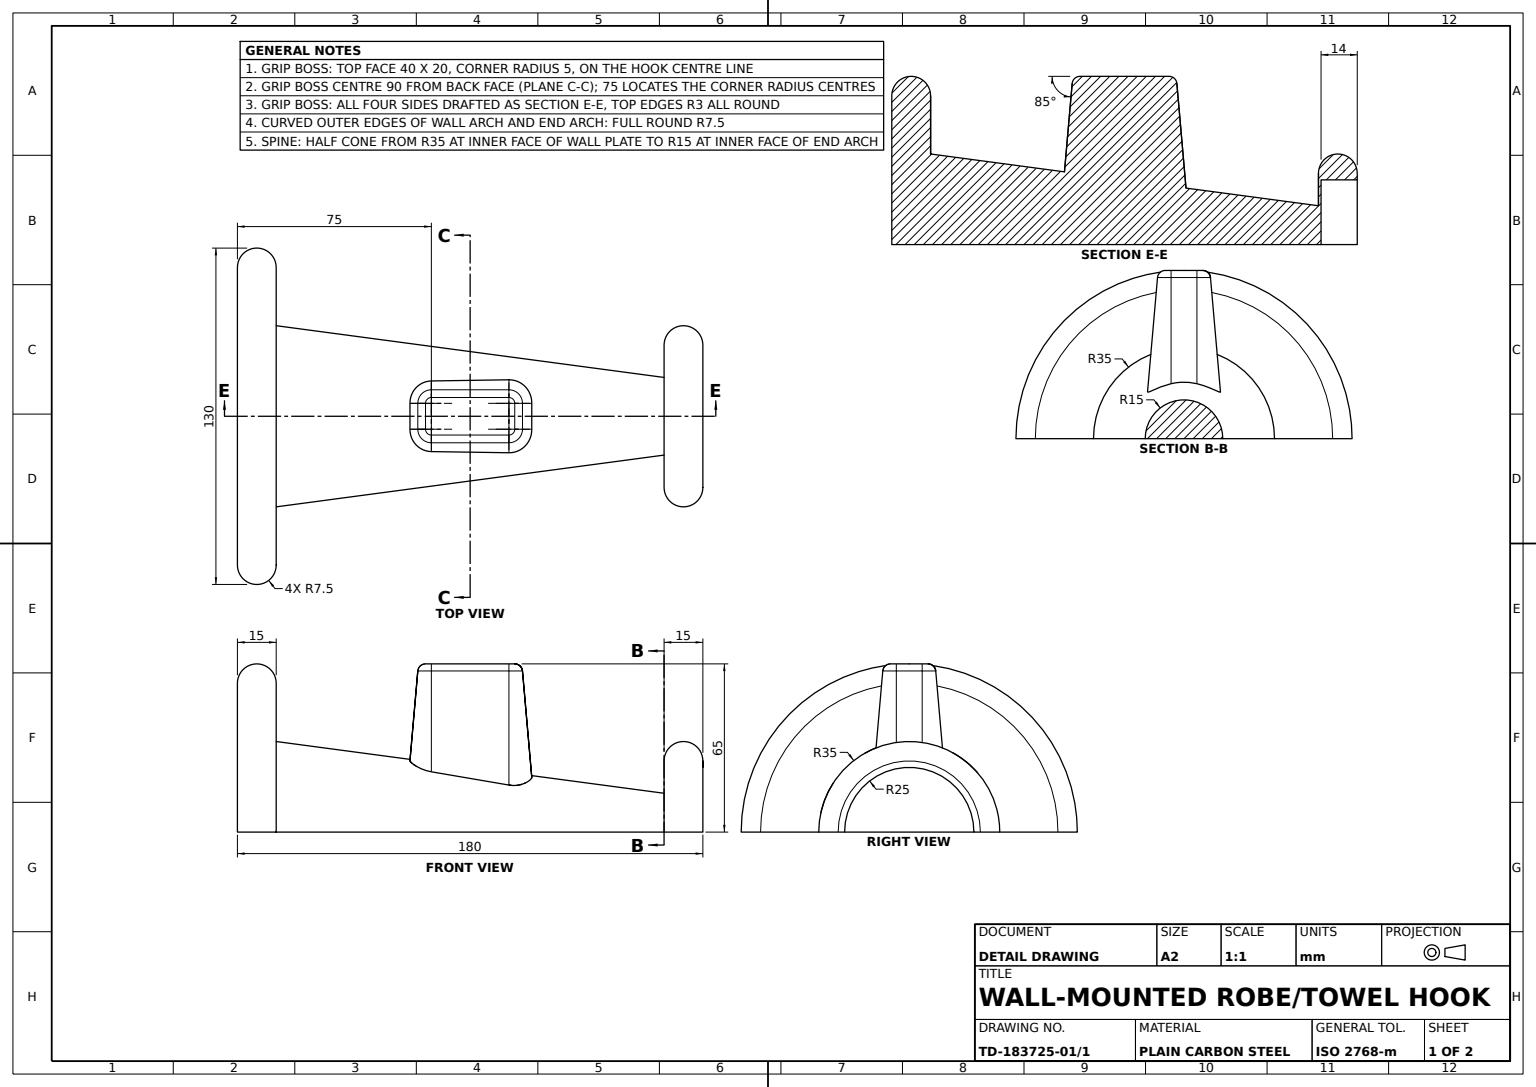
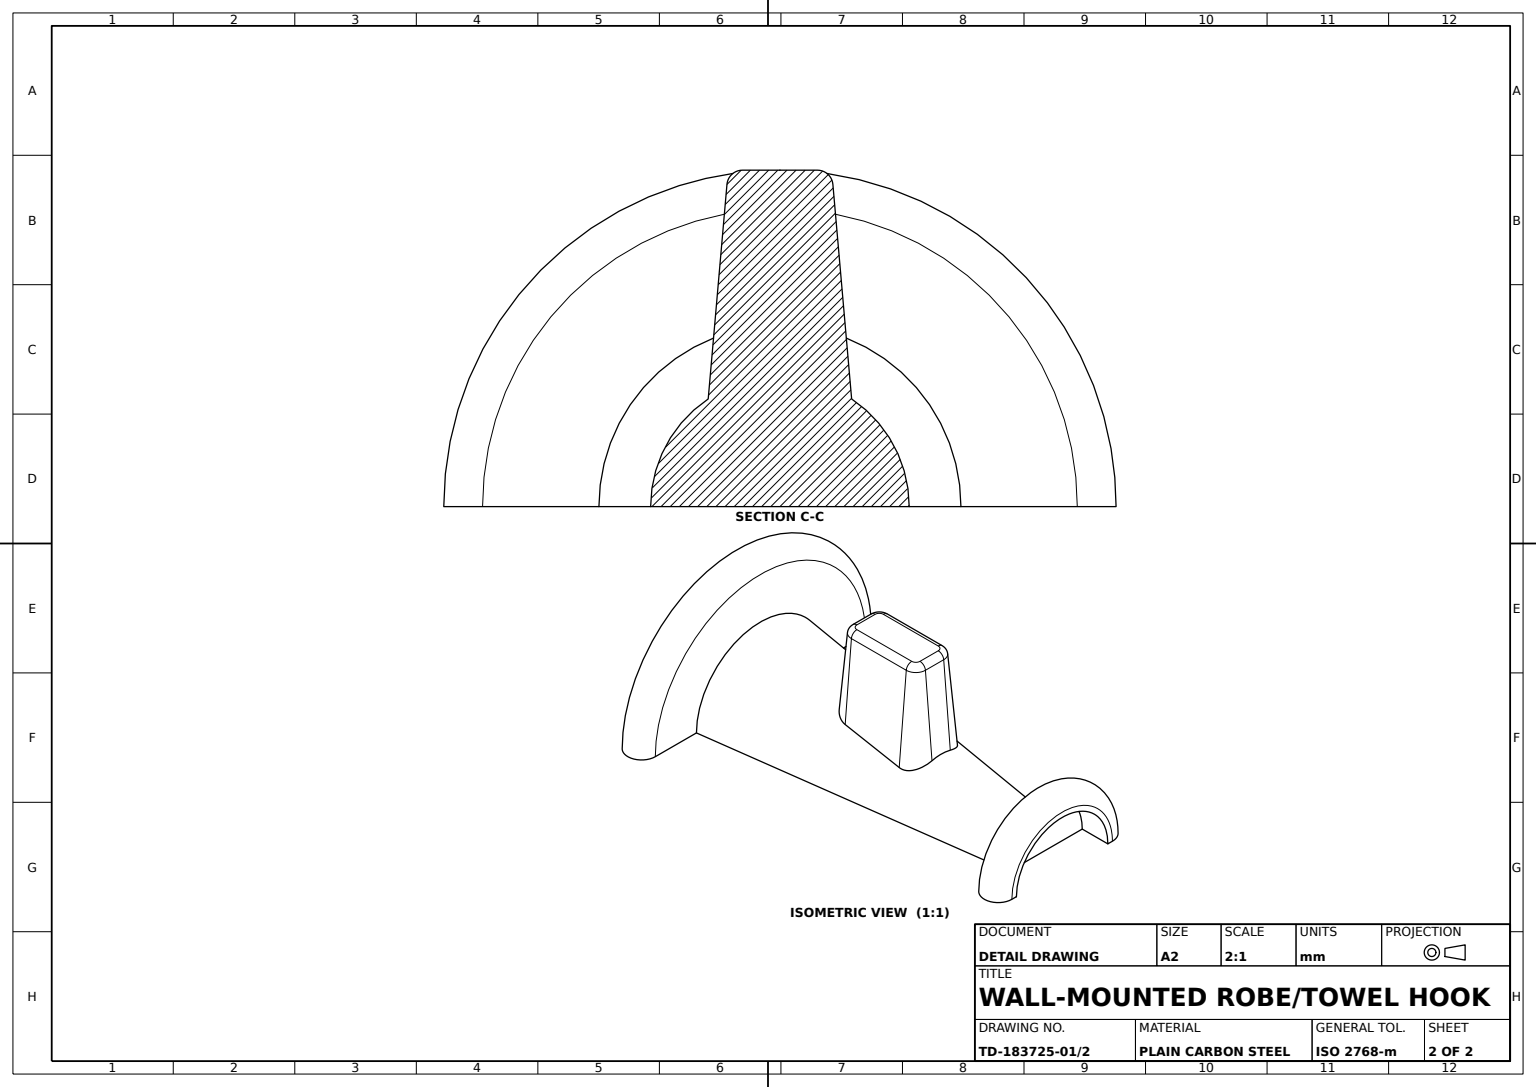
ISO-10303-21;
HEADER;
FILE_DESCRIPTION((''),'2;1');
FILE_NAME('','',(''),(''),'','','');
FILE_SCHEMA(('AUTOMOTIVE_DESIGN'));
ENDSEC;
DATA;
#1=APPLICATION_CONTEXT('');
#2=PRODUCT_CONTEXT('',#1,'mechanical');
#3=PRODUCT('','','',(#2));
#4=PRODUCT_DEFINITION_FORMATION('','',#3);
#5=PRODUCT_DEFINITION_CONTEXT('',#1,'design');
#6=PRODUCT_DEFINITION('','',#4,#5);
#7=PRODUCT_DEFINITION_SHAPE('','',#6);
#8=(LENGTH_UNIT()NAMED_UNIT(*)SI_UNIT(.MILLI.,.METRE.));
#9=(NAMED_UNIT(*)PLANE_ANGLE_UNIT()SI_UNIT($,.RADIAN.));
#10=(NAMED_UNIT(*)SI_UNIT($,.STERADIAN.)SOLID_ANGLE_UNIT());
#11=UNCERTAINTY_MEASURE_WITH_UNIT(LENGTH_MEASURE(1.E-05),#8,'distance_accuracy_value','');
#12=(GEOMETRIC_REPRESENTATION_CONTEXT(3)GLOBAL_UNCERTAINTY_ASSIGNED_CONTEXT((#11))GLOBAL_UNIT_ASSIGNED_CONTEXT((#8,#9,#10))REPRESENTATION_CONTEXT('',''));
#13=CARTESIAN_POINT('',(-90.,0.,-57.5));
#14=VERTEX_POINT('',#13);
#15=CARTESIAN_POINT('',(-90.,0.,57.5));
#16=VERTEX_POINT('',#15);
#17=CARTESIAN_POINT('',(-90.,0.,0.));
#18=DIRECTION('',(0.,0.,1.));
#19=VECTOR('',#18,1000.);
#20=LINE('',#17,#19);
#21=EDGE_CURVE('',#14,#16,#20,.T.);
#22=ORIENTED_EDGE('',*,*,#21,.T.);
#23=DIRECTION('',(-1.,0.,0.));
#24=AXIS2_PLACEMENT_3D('',#17,#23,#18);
#25=CIRCLE('',#24,57.5);
#26=EDGE_CURVE('',#16,#14,#25,.T.);
#27=ORIENTED_EDGE('',*,*,#26,.T.);
#28=EDGE_LOOP('',(#22,#27));
#29=FACE_OUTER_BOUND('',#28,.T.);
#30=PLANE('',#24);
#31=ADVANCED_FACE('',(#29),#30,.T.);
#32=CARTESIAN_POINT('',(15.,62.261467,-10.239591));
#33=VERTEX_POINT('',#32);
#34=CARTESIAN_POINT('',(20.239591,62.261467,-5.));
#35=VERTEX_POINT('',#34);
#36=CARTESIAN_POINT('',(15.,62.261467,-5.));
#37=DIRECTION('',(0.,-1.,0.));
#38=DIRECTION('',(0.,0.,-1.));
#39=AXIS2_PLACEMENT_3D('',#36,#37,#38);
#40=CIRCLE('',#39,5.239591);
#41=EDGE_CURVE('',#33,#35,#40,.T.);
#42=ORIENTED_EDGE('',*,*,#41,.F.);
#43=CARTESIAN_POINT('',(15.,65.,-7.251006));
#44=VERTEX_POINT('',#43);
#45=CARTESIAN_POINT('',(15.,62.,-7.251006));
#46=DIRECTION('',(1.,0.,0.));
#47=AXIS2_PLACEMENT_3D('',#45,#46,#38);
#48=CIRCLE('',#47,3.);
#49=EDGE_CURVE('',#33,#44,#48,.T.);
#50=ORIENTED_EDGE('',*,*,#49,.T.);
#51=CARTESIAN_POINT('',(17.251006,65.,-5.));
#52=VERTEX_POINT('',#51);
#53=CARTESIAN_POINT('',(15.,65.,-5.));
#54=DIRECTION('',(0.,1.,0.));
#55=AXIS2_PLACEMENT_3D('',#53,#54,#38);
#56=CIRCLE('',#55,2.251006);
#57=EDGE_CURVE('',#52,#44,#56,.T.);
#58=ORIENTED_EDGE('',*,*,#57,.F.);
#59=CARTESIAN_POINT('',(17.251006,62.,-5.));
#60=AXIS2_PLACEMENT_3D('',#59,#18,#46);
#61=CIRCLE('',#60,3.);
#62=EDGE_CURVE('',#35,#52,#61,.T.);
#63=ORIENTED_EDGE('',*,*,#62,.F.);
#64=EDGE_LOOP('',(#42,#50,#58,#63));
#65=FACE_OUTER_BOUND('',#64,.T.);
#66=CARTESIAN_POINT('',(15.,62.,-5.));
#67=AXIS2_PLACEMENT_3D('',#66,#37,#38);
#68=TOROIDAL_SURFACE('',#67,2.251006,3.);
#69=ADVANCED_FACE('',(#65),#68,.T.);
#70=CARTESIAN_POINT('',(-17.251006,65.,5.));
#71=VERTEX_POINT('',#70);
#72=CARTESIAN_POINT('',(-20.239591,62.261467,5.));
#73=VERTEX_POINT('',#72);
#74=CARTESIAN_POINT('',(-17.251006,62.,5.));
#75=AXIS2_PLACEMENT_3D('',#74,#18,#46);
#76=CIRCLE('',#75,3.);
#77=EDGE_CURVE('',#71,#73,#76,.T.);
#78=ORIENTED_EDGE('',*,*,#77,.F.);
#79=CARTESIAN_POINT('',(-17.251006,65.,-5.));
#80=VERTEX_POINT('',#79);
#81=LINE('',#70,#19);
#82=EDGE_CURVE('',#80,#71,#81,.T.);
#83=ORIENTED_EDGE('',*,*,#82,.F.);
#84=CARTESIAN_POINT('',(-20.239591,62.261467,-5.));
#85=VERTEX_POINT('',#84);
#86=CARTESIAN_POINT('',(-17.251006,62.,-5.));
#87=AXIS2_PLACEMENT_3D('',#86,#18,#46);
#88=CIRCLE('',#87,3.);
#89=EDGE_CURVE('',#80,#85,#88,.T.);
#90=ORIENTED_EDGE('',*,*,#89,.T.);
#91=VECTOR('',#38,1000.);
#92=LINE('',#84,#91);
#93=EDGE_CURVE('',#73,#85,#92,.T.);
#94=ORIENTED_EDGE('',*,*,#93,.F.);
#95=EDGE_LOOP('',(#78,#83,#90,#94));
#96=FACE_OUTER_BOUND('',#95,.T.);
#97=AXIS2_PLACEMENT_3D('',#86,#38,#23);
#98=CYLINDRICAL_SURFACE('',#97,3.);
#99=ADVANCED_FACE('',(#96),#98,.T.);
#100=CARTESIAN_POINT('',(76.,0.,-25.));
#101=VERTEX_POINT('',#100);
#102=CARTESIAN_POINT('',(76.,0.,25.));
#103=VERTEX_POINT('',#102);
#104=CARTESIAN_POINT('',(76.,0.,94.));
#105=LINE('',#104,#19);
#106=EDGE_CURVE('',#101,#103,#105,.T.);
#107=ORIENTED_EDGE('',*,*,#106,.F.);
#108=CARTESIAN_POINT('',(76.,0.,0.));
#109=AXIS2_PLACEMENT_3D('',#108,#46,#38);
#110=CIRCLE('',#109,25.);
#111=EDGE_CURVE('',#101,#103,#110,.T.);
#112=ORIENTED_EDGE('',*,*,#111,.T.);
#113=EDGE_LOOP('',(#107,#112));
#114=FACE_OUTER_BOUND('',#113,.T.);
#115=PLANE('',#109);
#116=ADVANCED_FACE('',(#114),#115,.T.);
#117=CARTESIAN_POINT('',(23.828296,21.24238,5.));
#118=VERTEX_POINT('',#117);
#119=CARTESIAN_POINT('',(20.239591,62.261467,5.));
#120=VERTEX_POINT('',#119);
#121=CARTESIAN_POINT('',(20.,65.,5.));
#122=DIRECTION('',(-0.087155743,0.996194698,0.));
#123=VECTOR('',#122,1000.);
#124=LINE('',#121,#123);
#125=EDGE_CURVE('',#118,#120,#124,.T.);
#126=ORIENTED_EDGE('',*,*,#125,.T.);
#127=CARTESIAN_POINT('',(15.,62.261467,10.239591));
#128=VERTEX_POINT('',#127);
#129=CARTESIAN_POINT('',(15.,62.261467,5.));
#130=AXIS2_PLACEMENT_3D('',#129,#37,#38);
#131=CIRCLE('',#130,5.239591);
#132=EDGE_CURVE('',#120,#128,#131,.T.);
#133=ORIENTED_EDGE('',*,*,#132,.T.);
#134=CARTESIAN_POINT('',(15.,18.173632,14.096776));
#135=VERTEX_POINT('',#134);
#136=CARTESIAN_POINT('',(15.,65.,10.));
#137=DIRECTION('',(0.,0.996194698,-0.087155743));
#138=VECTOR('',#137,1000.);
#139=LINE('',#136,#138);
#140=EDGE_CURVE('',#135,#128,#139,.T.);
#141=ORIENTED_EDGE('',*,*,#140,.F.);
#142=CARTESIAN_POINT('',(23.840601,21.101725,5.590409));
#143=CARTESIAN_POINT('',(23.795702,20.944319,6.174844));
#144=CARTESIAN_POINT('',(23.643977,20.683423,7.042667));
#145=CARTESIAN_POINT('',(23.579195,20.592513,7.329711));
#146=CARTESIAN_POINT('',(23.424423,20.406792,7.889331));
#147=CARTESIAN_POINT('',(23.334202,20.311543,8.163393));
#148=CARTESIAN_POINT('',(23.128661,20.117169,8.700562));
#149=CARTESIAN_POINT('',(23.013343,20.018041,8.963668));
#150=CARTESIAN_POINT('',(22.757306,19.816981,9.479197));
#151=CARTESIAN_POINT('',(22.615811,19.714543,9.73281));
#152=CARTESIAN_POINT('',(22.157707,19.409162,10.467784));
#153=CARTESIAN_POINT('',(21.809445,19.208631,10.922403));
#154=CARTESIAN_POINT('',(21.220199,18.923437,11.553938));
#155=CARTESIAN_POINT('',(21.01254,18.831012,11.755982));
#156=CARTESIAN_POINT('',(20.572849,18.654017,12.142651));
#157=CARTESIAN_POINT('',(20.340224,18.569371,12.327468));
#158=CARTESIAN_POINT('',(19.619318,18.337421,12.842278));
#159=CARTESIAN_POINT('',(19.103668,18.20966,13.137737));
#160=CARTESIAN_POINT('',(18.269214,18.077938,13.503422));
#161=CARTESIAN_POINT('',(17.98184,18.04451,13.611482));
#162=CARTESIAN_POINT('',(17.403424,18.002399,13.794297));
#163=CARTESIAN_POINT('',(17.110364,17.993364,13.869986));
#164=CARTESIAN_POINT('',(16.516526,18.000652,13.989928));
#165=CARTESIAN_POINT('',(16.215749,18.016974,14.034185));
#166=CARTESIAN_POINT('',(15.606218,18.076326,14.09024));
#167=CARTESIAN_POINT('',(15.300917,18.119158,14.101542));
#168=B_SPLINE_CURVE_WITH_KNOTS('',3,(#117,#142,#143,#144,#145,#146,#147,#148,#149,#150,#151,#152,#153,#154,#155,#156,#157,#158,#159,#160,#161,#162,#163,#164,#165,#166,#167,#134),.UNSPECIFIED.,.F.,.F.,(4,2,2,2,2,2,2,2,2,2,2,2,2,4),(0.001090919,0.002909668,0.003819042,0.004728417,0.005637791,0.006547165,0.008365914,0.009275289,0.010184663,0.012003412,0.012912786,0.013822161,0.014731535,0.01564091),.UNSPECIFIED.);
#169=EDGE_CURVE('',#118,#135,#168,.T.);
#170=ORIENTED_EDGE('',*,*,#169,.F.);
#171=EDGE_LOOP('',(#126,#133,#141,#170));
#172=FACE_OUTER_BOUND('',#171,.T.);
#173=CARTESIAN_POINT('',(15.,65.,5.));
#174=AXIS2_PLACEMENT_3D('',#173,#37,#18);
#175=CONICAL_SURFACE('',#174,5.,0.087266463);
#176=ADVANCED_FACE('',(#172),#175,.T.);
#177=CARTESIAN_POINT('',(90.,0.,-25.));
#178=VERTEX_POINT('',#177);
#179=CARTESIAN_POINT('',(90.,0.,25.));
#180=VERTEX_POINT('',#179);
#181=CARTESIAN_POINT('',(90.,0.,0.));
#182=AXIS2_PLACEMENT_3D('',#181,#46,#38);
#183=CIRCLE('',#182,25.);
#184=EDGE_CURVE('',#178,#180,#183,.T.);
#185=ORIENTED_EDGE('',*,*,#184,.T.);
#186=VECTOR('',#23,1000.);
#187=LINE('',#102,#186);
#188=EDGE_CURVE('',#180,#103,#187,.T.);
#189=ORIENTED_EDGE('',*,*,#188,.T.);
#190=ORIENTED_EDGE('',*,*,#111,.F.);
#191=VECTOR('',#46,1000.);
#192=LINE('',#100,#191);
#193=EDGE_CURVE('',#101,#178,#192,.T.);
#194=ORIENTED_EDGE('',*,*,#193,.T.);
#195=EDGE_LOOP('',(#185,#189,#190,#194));
#196=FACE_OUTER_BOUND('',#195,.T.);
#197=CYLINDRICAL_SURFACE('',#109,25.);
#198=ADVANCED_FACE('',(#196),#197,.F.);
#199=CARTESIAN_POINT('',(-75.,0.,57.5));
#200=VERTEX_POINT('',#199);
#201=CARTESIAN_POINT('',(-75.,0.,-57.5));
#202=VERTEX_POINT('',#201);
#203=CARTESIAN_POINT('',(-75.,0.,0.));
#204=AXIS2_PLACEMENT_3D('',#203,#23,#18);
#205=CIRCLE('',#204,57.5);
#206=EDGE_CURVE('',#200,#202,#205,.T.);
#207=ORIENTED_EDGE('',*,*,#206,.T.);
#208=CARTESIAN_POINT('',(-82.5,0.,-57.5));
#209=AXIS2_PLACEMENT_3D('',#208,#37,#38);
#210=CIRCLE('',#209,7.5);
#211=EDGE_CURVE('',#14,#202,#210,.T.);
#212=ORIENTED_EDGE('',*,*,#211,.F.);
#213=ORIENTED_EDGE('',*,*,#26,.F.);
#214=CARTESIAN_POINT('',(-82.5,0.,57.5));
#215=AXIS2_PLACEMENT_3D('',#214,#37,#38);
#216=CIRCLE('',#215,7.5);
#217=EDGE_CURVE('',#200,#16,#216,.T.);
#218=ORIENTED_EDGE('',*,*,#217,.F.);
#219=EDGE_LOOP('',(#207,#212,#213,#218));
#220=FACE_OUTER_BOUND('',#219,.T.);
#221=CARTESIAN_POINT('',(-82.5,0.,0.));
#222=AXIS2_PLACEMENT_3D('',#221,#23,#18);
#223=TOROIDAL_SURFACE('',#222,57.5,7.5);
#224=ADVANCED_FACE('',(#220),#223,.T.);
#225=CARTESIAN_POINT('',(-15.,23.296257,13.648605));
#226=VERTEX_POINT('',#225);
#227=CARTESIAN_POINT('',(-23.267357,27.653934,5.));
#228=VERTEX_POINT('',#227);
#229=CARTESIAN_POINT('',(-15.286863,23.342981,13.644517));
#230=CARTESIAN_POINT('',(-15.571632,23.39812,13.625462));
#231=CARTESIAN_POINT('',(-16.13718,23.524275,13.55813));
#232=CARTESIAN_POINT('',(-16.419535,23.595752,13.509462));
#233=CARTESIAN_POINT('',(-17.24849,23.829231,13.322204));
#234=CARTESIAN_POINT('',(-17.773834,24.008665,13.144495));
#235=CARTESIAN_POINT('',(-18.526695,24.303572,12.805119));
#236=CARTESIAN_POINT('',(-18.772818,24.406707,12.679069));
#237=CARTESIAN_POINT('',(-19.247498,24.617633,12.405792));
#238=CARTESIAN_POINT('',(-19.475861,24.725257,12.258861));
#239=CARTESIAN_POINT('',(-20.135824,25.052517,11.788166));
#240=CARTESIAN_POINT('',(-20.542582,25.276497,11.43483));
#241=CARTESIAN_POINT('',(-21.291765,25.726959,10.645748));
#242=CARTESIAN_POINT('',(-21.623823,25.947177,10.220874));
#243=CARTESIAN_POINT('',(-22.060957,26.264462,9.537608));
#244=CARTESIAN_POINT('',(-22.196427,26.36806,9.302129));
#245=CARTESIAN_POINT('',(-22.446305,26.570013,8.814918));
#246=CARTESIAN_POINT('',(-22.561252,26.668877,8.561765));
#247=CARTESIAN_POINT('',(-22.868248,26.952116,7.786987));
#248=CARTESIAN_POINT('',(-23.022121,27.122148,7.253806));
#249=CARTESIAN_POINT('',(-23.175243,27.346177,6.427897));
#250=CARTESIAN_POINT('',(-23.21324,27.41567,6.148213));
#251=CARTESIAN_POINT('',(-23.261622,27.543614,5.579548));
#252=CARTESIAN_POINT('',(-23.271881,27.602225,5.28938));
#253=B_SPLINE_CURVE_WITH_KNOTS('',3,(#225,#229,#230,#231,#232,#233,#234,#235,#236,#237,#238,#239,#240,#241,#242,#243,#244,#245,#246,#247,#248,#249,#250,#251,#252,#227),.UNSPECIFIED.,.F.,.F.,(4,2,2,2,2,2,2,2,2,2,2,2,4),(0.001072727,0.001944374,0.00281602,0.004559313,0.005430959,0.006302605,0.008045898,0.00978919,0.010660837,0.011532483,0.013275776,0.014147422,0.015019068),.UNSPECIFIED.);
#254=EDGE_CURVE('',#226,#228,#253,.T.);
#255=ORIENTED_EDGE('',*,*,#254,.F.);
#256=CARTESIAN_POINT('',(-15.,62.261467,10.239591));
#257=VERTEX_POINT('',#256);
#258=CARTESIAN_POINT('',(-15.,65.,10.));
#259=LINE('',#258,#138);
#260=EDGE_CURVE('',#226,#257,#259,.T.);
#261=ORIENTED_EDGE('',*,*,#260,.T.);
#262=CARTESIAN_POINT('',(-15.,62.261467,5.));
#263=AXIS2_PLACEMENT_3D('',#262,#37,#38);
#264=CIRCLE('',#263,5.239591);
#265=EDGE_CURVE('',#257,#73,#264,.T.);
#266=ORIENTED_EDGE('',*,*,#265,.T.);
#267=CARTESIAN_POINT('',(-20.,65.,5.));
#268=DIRECTION('',(0.087155743,0.996194698,0.));
#269=VECTOR('',#268,1000.);
#270=LINE('',#267,#269);
#271=EDGE_CURVE('',#228,#73,#270,.T.);
#272=ORIENTED_EDGE('',*,*,#271,.F.);
#273=EDGE_LOOP('',(#255,#261,#266,#272));
#274=FACE_OUTER_BOUND('',#273,.T.);
#275=CARTESIAN_POINT('',(-15.,65.,5.));
#276=AXIS2_PLACEMENT_3D('',#275,#37,#18);
#277=CONICAL_SURFACE('',#276,5.,0.087266463);
#278=ADVANCED_FACE('',(#274),#277,.T.);
#279=CARTESIAN_POINT('',(-15.,23.296257,-13.648605));
#280=VERTEX_POINT('',#279);
#281=CARTESIAN_POINT('',(-15.,62.261467,-10.239591));
#282=VERTEX_POINT('',#281);
#283=CARTESIAN_POINT('',(-15.,65.,-10.));
#284=DIRECTION('',(0.,0.996194698,0.087155743));
#285=VECTOR('',#284,1000.);
#286=LINE('',#283,#285);
#287=EDGE_CURVE('',#280,#282,#286,.T.);
#288=ORIENTED_EDGE('',*,*,#287,.T.);
#289=LINE('',#32,#191);
#290=EDGE_CURVE('',#282,#33,#289,.T.);
#291=ORIENTED_EDGE('',*,*,#290,.T.);
#292=CARTESIAN_POINT('',(15.,18.173632,-14.096776));
#293=VERTEX_POINT('',#292);
#294=CARTESIAN_POINT('',(15.,65.,-10.));
#295=LINE('',#294,#285);
#296=EDGE_CURVE('',#293,#33,#295,.T.);
#297=ORIENTED_EDGE('',*,*,#296,.F.);
#298=CARTESIAN_POINT('',(-9.99341,22.480784,-13.719949));
#299=CARTESIAN_POINT('',(-4.989326,21.650749,-13.792568));
#300=CARTESIAN_POINT('',(5.011643,19.94884,-13.941466));
#301=CARTESIAN_POINT('',(10.008571,19.077218,-14.017723));
#302=B_SPLINE_CURVE_WITH_KNOTS('',3,(#279,#298,#299,#300,#301,#292),.UNSPECIFIED.,.F.,.F.,(4,2,4),(0.000000203,0.015218959,0.030437715),.UNSPECIFIED.);
#303=EDGE_CURVE('',#280,#293,#302,.T.);
#304=ORIENTED_EDGE('',*,*,#303,.F.);
#305=EDGE_LOOP('',(#288,#291,#297,#304));
#306=FACE_OUTER_BOUND('',#305,.T.);
#307=DIRECTION('',(0.,0.087155743,-0.996194698));
#308=AXIS2_PLACEMENT_3D('',#283,#307,#284);
#309=PLANE('',#308);
#310=ADVANCED_FACE('',(#306),#309,.T.);
#311=ORIENTED_EDGE('',*,*,#140,.T.);
#312=LINE('',#256,#186);
#313=EDGE_CURVE('',#128,#257,#312,.T.);
#314=ORIENTED_EDGE('',*,*,#313,.T.);
#315=ORIENTED_EDGE('',*,*,#260,.F.);
#316=CARTESIAN_POINT('',(10.008571,19.077218,14.017723));
#317=CARTESIAN_POINT('',(5.011643,19.94884,13.941466));
#318=CARTESIAN_POINT('',(-4.989326,21.650749,13.792568));
#319=CARTESIAN_POINT('',(-9.99341,22.480784,13.719949));
#320=B_SPLINE_CURVE_WITH_KNOTS('',3,(#134,#316,#317,#318,#319,#225),.UNSPECIFIED.,.F.,.F.,(4,2,4),(0.000000203,0.015218959,0.030437715),.UNSPECIFIED.);
#321=EDGE_CURVE('',#135,#226,#320,.T.);
#322=ORIENTED_EDGE('',*,*,#321,.F.);
#323=EDGE_LOOP('',(#311,#314,#315,#322));
#324=FACE_OUTER_BOUND('',#323,.T.);
#325=DIRECTION('',(0.,0.087155743,0.996194698));
#326=DIRECTION('',(0.,-0.996194698,0.087155743));
#327=AXIS2_PLACEMENT_3D('',#258,#325,#326);
#328=PLANE('',#327);
#329=ADVANCED_FACE('',(#324),#328,.T.);
#330=CARTESIAN_POINT('',(75.,0.,27.5));
#331=VERTEX_POINT('',#330);
#332=CARTESIAN_POINT('',(75.,0.,-27.5));
#333=VERTEX_POINT('',#332);
#334=CARTESIAN_POINT('',(75.,0.,0.));
#335=AXIS2_PLACEMENT_3D('',#334,#23,#18);
#336=CIRCLE('',#335,27.5);
#337=EDGE_CURVE('',#331,#333,#336,.T.);
#338=ORIENTED_EDGE('',*,*,#337,.F.);
#339=CARTESIAN_POINT('',(90.,0.,27.5));
#340=VERTEX_POINT('',#339);
#341=CARTESIAN_POINT('',(82.5,0.,27.5));
#342=AXIS2_PLACEMENT_3D('',#341,#37,#38);
#343=CIRCLE('',#342,7.5);
#344=EDGE_CURVE('',#340,#331,#343,.T.);
#345=ORIENTED_EDGE('',*,*,#344,.F.);
#346=CARTESIAN_POINT('',(90.,0.,-27.5));
#347=VERTEX_POINT('',#346);
#348=AXIS2_PLACEMENT_3D('',#181,#23,#18);
#349=CIRCLE('',#348,27.5);
#350=EDGE_CURVE('',#340,#347,#349,.T.);
#351=ORIENTED_EDGE('',*,*,#350,.T.);
#352=CARTESIAN_POINT('',(82.5,0.,-27.5));
#353=AXIS2_PLACEMENT_3D('',#352,#37,#38);
#354=CIRCLE('',#353,7.5);
#355=EDGE_CURVE('',#333,#347,#354,.T.);
#356=ORIENTED_EDGE('',*,*,#355,.F.);
#357=EDGE_LOOP('',(#338,#345,#351,#356));
#358=FACE_OUTER_BOUND('',#357,.T.);
#359=CARTESIAN_POINT('',(82.5,0.,0.));
#360=AXIS2_PLACEMENT_3D('',#359,#23,#18);
#361=TOROIDAL_SURFACE('',#360,27.5,7.5);
#362=ADVANCED_FACE('',(#358),#361,.T.);
#363=ORIENTED_EDGE('',*,*,#62,.T.);
#364=CARTESIAN_POINT('',(17.251006,65.,5.));
#365=VERTEX_POINT('',#364);
#366=LINE('',#51,#91);
#367=EDGE_CURVE('',#365,#52,#366,.T.);
#368=ORIENTED_EDGE('',*,*,#367,.F.);
#369=CARTESIAN_POINT('',(17.251006,62.,5.));
#370=AXIS2_PLACEMENT_3D('',#369,#18,#37);
#371=CIRCLE('',#370,3.);
#372=EDGE_CURVE('',#120,#365,#371,.T.);
#373=ORIENTED_EDGE('',*,*,#372,.F.);
#374=LINE('',#119,#19);
#375=EDGE_CURVE('',#35,#120,#374,.T.);
#376=ORIENTED_EDGE('',*,*,#375,.F.);
#377=EDGE_LOOP('',(#363,#368,#373,#376));
#378=FACE_OUTER_BOUND('',#377,.T.);
#379=CYLINDRICAL_SURFACE('',#60,3.);
#380=ADVANCED_FACE('',(#378),#379,.T.);
#381=ORIENTED_EDGE('',*,*,#337,.T.);
#382=CARTESIAN_POINT('',(75.,0.,-15.));
#383=VERTEX_POINT('',#382);
#384=LINE('',#334,#19);
#385=EDGE_CURVE('',#333,#383,#384,.T.);
#386=ORIENTED_EDGE('',*,*,#385,.T.);
#387=CARTESIAN_POINT('',(75.,0.,15.));
#388=VERTEX_POINT('',#387);
#389=CIRCLE('',#335,15.);
#390=EDGE_CURVE('',#388,#383,#389,.T.);
#391=ORIENTED_EDGE('',*,*,#390,.F.);
#392=EDGE_CURVE('',#388,#331,#384,.T.);
#393=ORIENTED_EDGE('',*,*,#392,.T.);
#394=EDGE_LOOP('',(#381,#386,#391,#393));
#395=FACE_OUTER_BOUND('',#394,.T.);
#396=PLANE('',#335);
#397=ADVANCED_FACE('',(#395),#396,.T.);
#398=ORIENTED_EDGE('',*,*,#184,.F.);
#399=LINE('',#181,#19);
#400=EDGE_CURVE('',#347,#178,#399,.T.);
#401=ORIENTED_EDGE('',*,*,#400,.F.);
#402=ORIENTED_EDGE('',*,*,#350,.F.);
#403=EDGE_CURVE('',#180,#340,#399,.T.);
#404=ORIENTED_EDGE('',*,*,#403,.F.);
#405=EDGE_LOOP('',(#398,#401,#402,#404));
#406=FACE_OUTER_BOUND('',#405,.T.);
#407=PLANE('',#348);
#408=ADVANCED_FACE('',(#406),#407,.F.);
#409=ORIENTED_EDGE('',*,*,#344,.T.);
#410=ORIENTED_EDGE('',*,*,#392,.F.);
#411=CARTESIAN_POINT('',(-75.,0.,35.));
#412=VERTEX_POINT('',#411);
#413=CARTESIAN_POINT('',(187.5,0.,0.));
#414=DIRECTION('',(0.991227901,0.,-0.13216372));
#415=VECTOR('',#414,1000.);
#416=LINE('',#413,#415);
#417=EDGE_CURVE('',#412,#388,#416,.T.);
#418=ORIENTED_EDGE('',*,*,#417,.F.);
#419=LINE('',#203,#19);
#420=EDGE_CURVE('',#412,#200,#419,.T.);
#421=ORIENTED_EDGE('',*,*,#420,.T.);
#422=ORIENTED_EDGE('',*,*,#217,.T.);
#423=ORIENTED_EDGE('',*,*,#21,.F.);
#424=ORIENTED_EDGE('',*,*,#211,.T.);
#425=CARTESIAN_POINT('',(-75.,0.,-35.));
#426=VERTEX_POINT('',#425);
#427=EDGE_CURVE('',#202,#426,#419,.T.);
#428=ORIENTED_EDGE('',*,*,#427,.T.);
#429=DIRECTION('',(-0.991227901,0.,-0.13216372));
#430=VECTOR('',#429,1000.);
#431=LINE('',#413,#430);
#432=EDGE_CURVE('',#383,#426,#431,.T.);
#433=ORIENTED_EDGE('',*,*,#432,.F.);
#434=ORIENTED_EDGE('',*,*,#385,.F.);
#435=ORIENTED_EDGE('',*,*,#355,.T.);
#436=ORIENTED_EDGE('',*,*,#400,.T.);
#437=ORIENTED_EDGE('',*,*,#193,.F.);
#438=ORIENTED_EDGE('',*,*,#106,.T.);
#439=ORIENTED_EDGE('',*,*,#188,.F.);
#440=ORIENTED_EDGE('',*,*,#403,.T.);
#441=EDGE_LOOP('',(#409,#410,#418,#421,#422,#423,#424,#428,#433,#434,#435,#436,#437,#438,#439,#440));
#442=FACE_OUTER_BOUND('',#441,.T.);
#443=CARTESIAN_POINT('',(-118.515789,0.,94.));
#444=AXIS2_PLACEMENT_3D('',#443,#37,#38);
#445=PLANE('',#444);
#446=ADVANCED_FACE('',(#442),#445,.T.);
#447=ORIENTED_EDGE('',*,*,#321,.T.);
#448=ORIENTED_EDGE('',*,*,#254,.T.);
#449=CARTESIAN_POINT('',(-23.267357,27.653934,-5.));
#450=VERTEX_POINT('',#449);
#451=CARTESIAN_POINT('',(-23.21552,28.246433,1.684171));
#452=CARTESIAN_POINT('',(-23.21552,28.246433,-1.684171));
#453=(BOUNDED_CURVE()B_SPLINE_CURVE(3,(#227,#451,#452,#449),.UNSPECIFIED.,.F.,.T.)B_SPLINE_CURVE_WITH_KNOTS((4,4),(2.964782726,3.318402581),.UNSPECIFIED.)CURVE()GEOMETRIC_REPRESENTATION_ITEM()RATIONAL_B_SPLINE_CURVE((1.,0.989606535,0.989606535,1.))REPRESENTATION_ITEM(''));
#454=EDGE_CURVE('',#228,#450,#453,.T.);
#455=ORIENTED_EDGE('',*,*,#454,.T.);
#456=CARTESIAN_POINT('',(-23.276303,27.551689,-5.572201));
#457=CARTESIAN_POINT('',(-23.228501,27.424407,-6.138968));
#458=CARTESIAN_POINT('',(-23.021567,27.12103,-7.258446));
#459=CARTESIAN_POINT('',(-22.865917,26.949872,-7.793344));
#460=CARTESIAN_POINT('',(-22.459244,26.574856,-8.818733));
#461=CARTESIAN_POINT('',(-22.205097,26.368921,-9.313037));
#462=CARTESIAN_POINT('',(-21.618695,25.943619,-10.228153));
#463=CARTESIAN_POINT('',(-21.286306,25.723568,-10.651891));
#464=CARTESIAN_POINT('',(-20.728199,25.388158,-11.239129));
#465=CARTESIAN_POINT('',(-20.531144,25.274931,-11.427563));
#466=CARTESIAN_POINT('',(-20.122439,25.051315,-11.782311));
#467=CARTESIAN_POINT('',(-19.910657,24.940786,-11.948974));
#468=CARTESIAN_POINT('',(-19.252704,24.614753,-12.417582));
#469=CARTESIAN_POINT('',(-18.784242,24.404669,-12.688544));
#470=CARTESIAN_POINT('',(-18.030411,24.109066,-13.029069));
#471=CARTESIAN_POINT('',(-17.769807,24.013656,-13.131561));
#472=CARTESIAN_POINT('',(-17.241926,23.835305,-13.308794));
#473=CARTESIAN_POINT('',(-16.973327,23.751806,-13.384221));
#474=CARTESIAN_POINT('',(-16.426269,23.597574,-13.508081));
#475=CARTESIAN_POINT('',(-16.147813,23.52684,-13.55652));
#476=CARTESIAN_POINT('',(-15.580182,23.39984,-13.624776));
#477=CARTESIAN_POINT('',(-15.289902,23.343476,-13.644474));
#478=B_SPLINE_CURVE_WITH_KNOTS('',3,(#449,#456,#457,#458,#459,#460,#461,#462,#463,#464,#465,#466,#467,#468,#469,#470,#471,#472,#473,#474,#475,#476,#477,#279),.UNSPECIFIED.,.F.,.F.,(4,2,2,2,2,2,2,2,2,2,2,4),(0.001078069,0.002820791,0.004563514,0.006306236,0.008048958,0.008920319,0.00979168,0.011534403,0.012405764,0.013277125,0.014148486,0.015019847),.UNSPECIFIED.);
#479=EDGE_CURVE('',#450,#280,#478,.T.);
#480=ORIENTED_EDGE('',*,*,#479,.T.);
#481=ORIENTED_EDGE('',*,*,#303,.T.);
#482=CARTESIAN_POINT('',(23.828296,21.24238,-5.));
#483=VERTEX_POINT('',#482);
#484=CARTESIAN_POINT('',(15.298841,18.119533,-14.101509));
#485=CARTESIAN_POINT('',(15.599827,18.077173,-14.090539));
#486=CARTESIAN_POINT('',(16.206404,18.017665,-14.035326));
#487=CARTESIAN_POINT('',(16.512197,18.000782,-13.990702));
#488=CARTESIAN_POINT('',(17.407913,17.98956,-13.810087));
#489=CARTESIAN_POINT('',(17.988074,18.03367,-13.626458));
#490=CARTESIAN_POINT('',(19.102691,18.209395,-13.138332));
#491=CARTESIAN_POINT('',(19.619347,18.337377,-12.842359));
#492=CARTESIAN_POINT('',(20.341704,18.569874,-12.326359));
#493=CARTESIAN_POINT('',(20.573954,18.654442,-12.141723));
#494=CARTESIAN_POINT('',(21.012914,18.831183,-11.755609));
#495=CARTESIAN_POINT('',(21.220838,18.92371,-11.553346));
#496=CARTESIAN_POINT('',(21.61503,19.114571,-11.130678));
#497=CARTESIAN_POINT('',(21.801294,19.212912,-10.910271));
#498=CARTESIAN_POINT('',(22.152678,19.413409,-10.450913));
#499=CARTESIAN_POINT('',(22.31765,19.515568,-10.211878));
#500=CARTESIAN_POINT('',(22.772841,19.819666,-9.47942));
#501=CARTESIAN_POINT('',(23.027145,20.020964,-8.966653));
#502=CARTESIAN_POINT('',(23.33594,20.31329,-8.158454));
#503=CARTESIAN_POINT('',(23.42696,20.409542,-7.881337));
#504=CARTESIAN_POINT('',(23.581941,20.596112,-7.318563));
#505=CARTESIAN_POINT('',(23.64553,20.685864,-7.034718));
#506=CARTESIAN_POINT('',(23.795218,20.943952,-6.175717));
#507=CARTESIAN_POINT('',(23.840658,21.101077,-5.593127));
#508=B_SPLINE_CURVE_WITH_KNOTS('',3,(#292,#484,#485,#486,#487,#488,#489,#490,#491,#492,#493,#494,#495,#496,#497,#498,#499,#500,#501,#502,#503,#504,#505,#506,#507,#482),.UNSPECIFIED.,.F.,.F.,(4,2,2,2,2,2,2,2,2,2,2,2,4),(0.001095531,0.002006676,0.002917821,0.004740111,0.006562401,0.007473546,0.008384691,0.009295836,0.010206981,0.012029271,0.012940416,0.013851561,0.015673851),.UNSPECIFIED.);
#509=EDGE_CURVE('',#293,#483,#508,.T.);
#510=ORIENTED_EDGE('',*,*,#509,.T.);
#511=CARTESIAN_POINT('',(23.759462,22.029153,-1.697471));
#512=CARTESIAN_POINT('',(23.759462,22.029153,1.697471));
#513=(BOUNDED_CURVE()B_SPLINE_CURVE(3,(#482,#511,#512,#117),.UNSPECIFIED.,.F.,.T.)B_SPLINE_CURVE_WITH_KNOTS((4,4),(6.049326624,6.51704399),.UNSPECIFIED.)CURVE()GEOMETRIC_REPRESENTATION_ITEM()RATIONAL_B_SPLINE_CURVE((1.,0.98185297,0.98185297,1.))REPRESENTATION_ITEM(''));
#514=EDGE_CURVE('',#483,#118,#513,.T.);
#515=ORIENTED_EDGE('',*,*,#514,.T.);
#516=ORIENTED_EDGE('',*,*,#169,.T.);
#517=EDGE_LOOP('',(#447,#448,#455,#480,#481,#510,#515,#516));
#518=FACE_BOUND('',#517,.T.);
#519=ORIENTED_EDGE('',*,*,#390,.T.);
#520=ORIENTED_EDGE('',*,*,#432,.T.);
#521=CIRCLE('',#204,35.);
#522=EDGE_CURVE('',#412,#426,#521,.T.);
#523=ORIENTED_EDGE('',*,*,#522,.F.);
#524=ORIENTED_EDGE('',*,*,#417,.T.);
#525=EDGE_LOOP('',(#519,#520,#523,#524));
#526=FACE_OUTER_BOUND('',#525,.T.);
#527=CONICAL_SURFACE('',#204,35.,0.132551532);
#528=ADVANCED_FACE('',(#518,#526),#527,.T.);
#529=CARTESIAN_POINT('',(15.,65.,7.251006));
#530=VERTEX_POINT('',#529);
#531=AXIS2_PLACEMENT_3D('',#173,#54,#38);
#532=CIRCLE('',#531,2.251006);
#533=EDGE_CURVE('',#530,#365,#532,.T.);
#534=ORIENTED_EDGE('',*,*,#533,.T.);
#535=ORIENTED_EDGE('',*,*,#367,.T.);
#536=ORIENTED_EDGE('',*,*,#57,.T.);
#537=CARTESIAN_POINT('',(-15.,65.,-7.251006));
#538=VERTEX_POINT('',#537);
#539=LINE('',#537,#186);
#540=EDGE_CURVE('',#44,#538,#539,.T.);
#541=ORIENTED_EDGE('',*,*,#540,.T.);
#542=CARTESIAN_POINT('',(-15.,65.,-5.));
#543=AXIS2_PLACEMENT_3D('',#542,#54,#38);
#544=CIRCLE('',#543,2.251006);
#545=EDGE_CURVE('',#538,#80,#544,.T.);
#546=ORIENTED_EDGE('',*,*,#545,.T.);
#547=ORIENTED_EDGE('',*,*,#82,.T.);
#548=CARTESIAN_POINT('',(-15.,65.,7.251006));
#549=VERTEX_POINT('',#548);
#550=AXIS2_PLACEMENT_3D('',#275,#54,#38);
#551=CIRCLE('',#550,2.251006);
#552=EDGE_CURVE('',#71,#549,#551,.T.);
#553=ORIENTED_EDGE('',*,*,#552,.T.);
#554=LINE('',#529,#191);
#555=EDGE_CURVE('',#549,#530,#554,.T.);
#556=ORIENTED_EDGE('',*,*,#555,.T.);
#557=EDGE_LOOP('',(#534,#535,#536,#541,#546,#547,#553,#556));
#558=FACE_OUTER_BOUND('',#557,.T.);
#559=AXIS2_PLACEMENT_3D('',#53,#37,#38);
#560=PLANE('',#559);
#561=ADVANCED_FACE('',(#558),#560,.F.);
#562=ORIENTED_EDGE('',*,*,#132,.F.);
#563=ORIENTED_EDGE('',*,*,#372,.T.);
#564=ORIENTED_EDGE('',*,*,#533,.F.);
#565=CARTESIAN_POINT('',(15.,62.,7.251006));
#566=AXIS2_PLACEMENT_3D('',#565,#46,#38);
#567=CIRCLE('',#566,3.);
#568=EDGE_CURVE('',#530,#128,#567,.T.);
#569=ORIENTED_EDGE('',*,*,#568,.T.);
#570=EDGE_LOOP('',(#562,#563,#564,#569));
#571=FACE_OUTER_BOUND('',#570,.T.);
#572=CARTESIAN_POINT('',(15.,62.,5.));
#573=AXIS2_PLACEMENT_3D('',#572,#37,#38);
#574=TOROIDAL_SURFACE('',#573,2.251006,3.);
#575=ADVANCED_FACE('',(#571),#574,.T.);
#576=CARTESIAN_POINT('',(-15.,62.261467,-5.));
#577=AXIS2_PLACEMENT_3D('',#576,#37,#38);
#578=CIRCLE('',#577,5.239591);
#579=EDGE_CURVE('',#85,#282,#578,.T.);
#580=ORIENTED_EDGE('',*,*,#579,.T.);
#581=ORIENTED_EDGE('',*,*,#287,.F.);
#582=ORIENTED_EDGE('',*,*,#479,.F.);
#583=CARTESIAN_POINT('',(-20.,65.,-5.));
#584=LINE('',#583,#269);
#585=EDGE_CURVE('',#450,#85,#584,.T.);
#586=ORIENTED_EDGE('',*,*,#585,.T.);
#587=EDGE_LOOP('',(#580,#581,#582,#586));
#588=FACE_OUTER_BOUND('',#587,.T.);
#589=AXIS2_PLACEMENT_3D('',#542,#37,#18);
#590=CONICAL_SURFACE('',#589,5.,0.087266463);
#591=ADVANCED_FACE('',(#588),#590,.T.);
#592=ORIENTED_EDGE('',*,*,#509,.F.);
#593=ORIENTED_EDGE('',*,*,#296,.T.);
#594=ORIENTED_EDGE('',*,*,#41,.T.);
#595=CARTESIAN_POINT('',(20.,65.,-5.));
#596=LINE('',#595,#123);
#597=EDGE_CURVE('',#483,#35,#596,.T.);
#598=ORIENTED_EDGE('',*,*,#597,.F.);
#599=EDGE_LOOP('',(#592,#593,#594,#598));
#600=FACE_OUTER_BOUND('',#599,.T.);
#601=CONICAL_SURFACE('',#559,5.,0.087266463);
#602=ADVANCED_FACE('',(#600),#601,.T.);
#603=ORIENTED_EDGE('',*,*,#313,.F.);
#604=ORIENTED_EDGE('',*,*,#568,.F.);
#605=ORIENTED_EDGE('',*,*,#555,.F.);
#606=CARTESIAN_POINT('',(-15.,62.,7.251006));
#607=AXIS2_PLACEMENT_3D('',#606,#46,#38);
#608=CIRCLE('',#607,3.);
#609=EDGE_CURVE('',#549,#257,#608,.T.);
#610=ORIENTED_EDGE('',*,*,#609,.T.);
#611=EDGE_LOOP('',(#603,#604,#605,#610));
#612=FACE_OUTER_BOUND('',#611,.T.);
#613=AXIS2_PLACEMENT_3D('',#565,#23,#18);
#614=CYLINDRICAL_SURFACE('',#613,3.);
#615=ADVANCED_FACE('',(#612),#614,.T.);
#616=ORIENTED_EDGE('',*,*,#49,.F.);
#617=ORIENTED_EDGE('',*,*,#290,.F.);
#618=CARTESIAN_POINT('',(-15.,62.,-7.251006));
#619=AXIS2_PLACEMENT_3D('',#618,#46,#38);
#620=CIRCLE('',#619,3.);
#621=EDGE_CURVE('',#282,#538,#620,.T.);
#622=ORIENTED_EDGE('',*,*,#621,.T.);
#623=ORIENTED_EDGE('',*,*,#540,.F.);
#624=EDGE_LOOP('',(#616,#617,#622,#623));
#625=FACE_OUTER_BOUND('',#624,.T.);
#626=CYLINDRICAL_SURFACE('',#47,3.);
#627=ADVANCED_FACE('',(#625),#626,.T.);
#628=ORIENTED_EDGE('',*,*,#545,.F.);
#629=ORIENTED_EDGE('',*,*,#621,.F.);
#630=ORIENTED_EDGE('',*,*,#579,.F.);
#631=ORIENTED_EDGE('',*,*,#89,.F.);
#632=EDGE_LOOP('',(#628,#629,#630,#631));
#633=FACE_OUTER_BOUND('',#632,.T.);
#634=CARTESIAN_POINT('',(-15.,62.,-5.));
#635=AXIS2_PLACEMENT_3D('',#634,#37,#38);
#636=TOROIDAL_SURFACE('',#635,2.251006,3.);
#637=ADVANCED_FACE('',(#633),#636,.T.);
#638=ORIENTED_EDGE('',*,*,#597,.T.);
#639=ORIENTED_EDGE('',*,*,#375,.T.);
#640=ORIENTED_EDGE('',*,*,#125,.F.);
#641=ORIENTED_EDGE('',*,*,#514,.F.);
#642=EDGE_LOOP('',(#638,#639,#640,#641));
#643=FACE_OUTER_BOUND('',#642,.T.);
#644=DIRECTION('',(0.996194698,0.087155743,0.));
#645=AXIS2_PLACEMENT_3D('',#595,#644,#122);
#646=PLANE('',#645);
#647=ADVANCED_FACE('',(#643),#646,.T.);
#648=ORIENTED_EDGE('',*,*,#454,.F.);
#649=ORIENTED_EDGE('',*,*,#271,.T.);
#650=ORIENTED_EDGE('',*,*,#93,.T.);
#651=ORIENTED_EDGE('',*,*,#585,.F.);
#652=EDGE_LOOP('',(#648,#649,#650,#651));
#653=FACE_OUTER_BOUND('',#652,.T.);
#654=DIRECTION('',(-0.996194698,0.087155743,0.));
#655=DIRECTION('',(-0.087155743,-0.996194698,0.));
#656=AXIS2_PLACEMENT_3D('',#583,#654,#655);
#657=PLANE('',#656);
#658=ADVANCED_FACE('',(#653),#657,.T.);
#659=ORIENTED_EDGE('',*,*,#206,.F.);
#660=ORIENTED_EDGE('',*,*,#420,.F.);
#661=ORIENTED_EDGE('',*,*,#522,.T.);
#662=ORIENTED_EDGE('',*,*,#427,.F.);
#663=EDGE_LOOP('',(#659,#660,#661,#662));
#664=FACE_OUTER_BOUND('',#663,.T.);
#665=PLANE('',#204);
#666=ADVANCED_FACE('',(#664),#665,.F.);
#667=ORIENTED_EDGE('',*,*,#609,.F.);
#668=ORIENTED_EDGE('',*,*,#552,.F.);
#669=ORIENTED_EDGE('',*,*,#77,.T.);
#670=ORIENTED_EDGE('',*,*,#265,.F.);
#671=EDGE_LOOP('',(#667,#668,#669,#670));
#672=FACE_OUTER_BOUND('',#671,.T.);
#673=CARTESIAN_POINT('',(-15.,62.,5.));
#674=AXIS2_PLACEMENT_3D('',#673,#37,#38);
#675=TOROIDAL_SURFACE('',#674,2.251006,3.);
#676=ADVANCED_FACE('',(#672),#675,.T.);
#677=CLOSED_SHELL('',(#31,#69,#99,#116,#176,#198,#224,#278,#310,#329,#362,#380,#397,#408,#446,#528,#561,#575,#591,#602,#615,#627,#637,#647,#658,#666,#676));
#678=MANIFOLD_SOLID_BREP('',#677);
#679=ADVANCED_BREP_SHAPE_REPRESENTATION('',(#678),#12);
#680=SHAPE_DEFINITION_REPRESENTATION(#7,#679);
ENDSEC;
END-ISO-10303-21;
